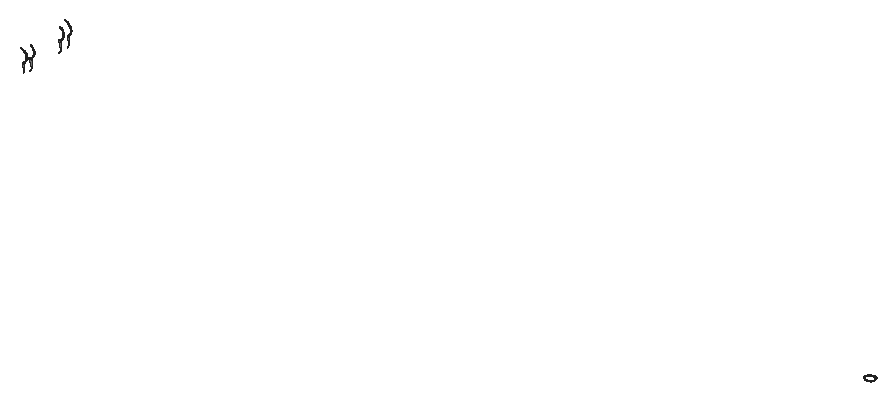
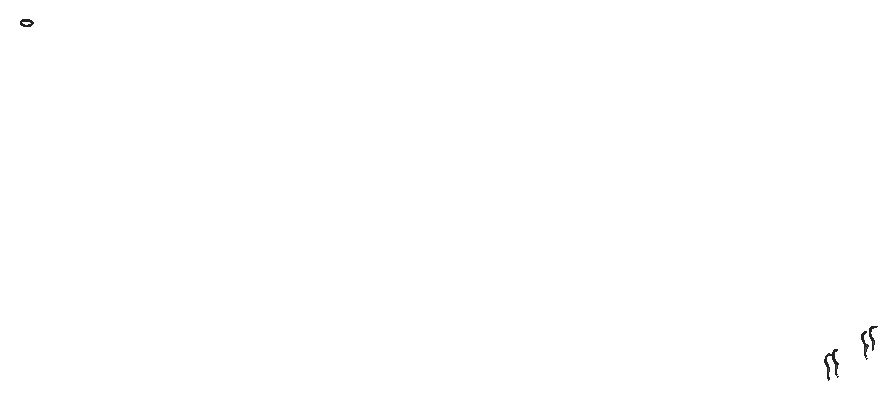
# SketchUp Ruby script. Lengths in inches.
U = 1.inch
M = Sketchup.active_model
def pt(a) = Geom::Point3d.new(a.map { |v| v * U })
def face(e, loops, mat)
  f = e.add_face(loops[0].map { |a| pt(a) })
  loops[1..].each { |l| e.add_face(l.map { |a| pt(a) }).erase! }
  f.material = f.back_material = mat if mat
  f
end
# faces: each face lists its corners as indices into pts; further lists are holes
def faces(e, pts, list, mat = nil) = list.each { |f| face(e, (f[0].is_a?(Array) ? f : [f]).map { |l| l.map { |i| pts[i] } }, mat) }
# xy, xz, yz: faces in a plane at the given z, y or x. An outline is a flat list of corners, or four numbers for a rectangle; further outlines are holes
def ring(l) = l.size == 4 ? [[l[0], l[1]], [l[2], l[1]], [l[2], l[3]], [l[0], l[3]]] : l.each_slice(2).to_a
def flat(e, list, mat, &to3) = list.each { |f| face(e, (f[0].is_a?(Array) ? f : [f]).map { |l| ring(l).map { |u, v| to3.(u, v) } }, mat) }
def xy(e, z, list, mat = nil) = flat(e, list, mat) { |x, y| [x, y, z] }
def xz(e, y, list, mat = nil) = flat(e, list, mat) { |x, z| [x, y, z] }
def yz(e, x, list, mat = nil) = flat(e, list, mat) { |y, z| [x, y, z] }
def lines(e, pts, list) = list.each { |a, b| e.add_line(pt(pts[a]), pt(pts[b])) }
# prism: a flat outline (further loops are holes) pulled along v
def prism(e, loops, v, mat = nil)
  f = face(e, loops, mat); d = Geom::Vector3d.new(v.map { |x| x * U })
  f.pushpull(f.normal.samedirection?(d) ? d.length : -d.length)
end
def box(e, o, s, mat = nil) = prism(e, [[o, [o[0] + s[0], o[1], o[2]], [o[0] + s[0], o[1] + s[1], o[2]], [o[0], o[1] + s[1], o[2]]]], [0, 0, s[2]], mat)
def at(x, y, z, deg = 0) = Geom::Transformation.translation(pt([x, y, z])) * Geom::Transformation.rotation(ORIGIN, Z_AXIS, deg.degrees)
def axes(o, x, y, z) = Geom::Transformation.new([*x, 0, *y, 0, *z, 0, *pt(o).to_a, 1])
def part(name) = M.definitions.add(name)
# library, detail: a bought-in or finely detailed component or shape, given as its bounding box
def library(name, o, s) = part(name).tap { |d| box(d.entities, o, s) }
def detail(e, o, s) = box(e.add_group.entities, o, s)
def put(e, d, t, mat = nil) = e.add_instance(d, t).tap { |i| i.material = mat if mat }
def group(e, t, mat = nil) = e.add_group.tap { |g| g.transformation = t; g.material = mat if mat }.entities
root = M.entities
M.materials.add("Material \#1").color = [140, 140, 140]
xy(root,30.4774,[[371.2232,117.1275,371.1558,117.1498,371.1662,117.166],[371.2232,117.1275,371.1662,117.166,371.2268,117.146],[371.2232,117.1275,371.2268,117.146,371.2948,117.1275],[371.2948,117.1275,371.2268,117.146,371.2912,117.146],[371.2948,117.1275,371.2912,117.146,371.3622,117.1498],
  [371.2912,117.146,371.3518,117.166,371.3622,117.1498],[371.1558,117.1498,371.101,117.1917,371.1168,117.2037],[371.1558,117.1498,371.1168,117.2037,371.1662,117.166],[371.3622,117.1498,371.3518,117.166,371.417,117.1917],[371.3518,117.166,371.4012,117.2037,371.417,117.1917],
  [371.101,117.1917,371.0651,117.2481,371.0845,117.2545],[371.101,117.1917,371.0845,117.2545,371.1168,117.2037],[371.417,117.1917,371.4012,117.2037,371.4529,117.2481],[371.4012,117.2037,371.4335,117.2545,371.4529,117.2481],[371.0651,117.2481,371.0527,117.3122,371.0733,117.3122],
  [371.0651,117.2481,371.0733,117.3122,371.0845,117.2545],[371.4529,117.2481,371.4335,117.2545,371.4653,117.3122],[371.4335,117.2545,371.4447,117.3122,371.4653,117.3122],[371.0527,117.3122,371.0651,117.3764,371.0845,117.37],[371.0527,117.3122,371.0845,117.37,371.0733,117.3122],
  [371.4447,117.3122,371.4335,117.37,371.4529,117.3764],[371.4447,117.3122,371.4529,117.3764,371.4653,117.3122],[371.0845,117.37,371.0651,117.3764,371.1168,117.4207],[371.4335,117.37,371.4012,117.4207,371.417,117.4328],[371.4335,117.37,371.417,117.4328,371.4529,117.3764],
  [371.0651,117.3764,371.101,117.4328,371.1168,117.4207],[371.1168,117.4207,371.101,117.4328,371.1662,117.4584],[371.4012,117.4207,371.3518,117.4584,371.3622,117.4746],[371.4012,117.4207,371.3622,117.4746,371.417,117.4328],[371.101,117.4328,371.1558,117.4746,371.1662,117.4584],
  [371.1662,117.4584,371.1558,117.4746,371.2268,117.4785],[371.3518,117.4584,371.2912,117.4784,371.2948,117.4969],[371.3518,117.4584,371.2948,117.4969,371.3622,117.4746],[371.1558,117.4746,371.2232,117.4969,371.2268,117.4785],[371.2912,117.4784,371.2232,117.4969,371.2948,117.4969],
  [371.2912,117.4784,371.2268,117.4785,371.2232,117.4969]],"Material \#1")
xy(root,30.4945,[[371.2232,117.1275,371.2268,117.146,371.1558,117.1498],[371.2232,117.1275,371.2912,117.146,371.2268,117.146],[371.2232,117.1275,371.2948,117.1275,371.2912,117.146],[371.2948,117.1275,371.3518,117.166,371.2912,117.146],[371.2948,117.1275,371.3622,117.1498,371.3518,117.166],
  [371.2268,117.146,371.1662,117.166,371.1558,117.1498],[371.1558,117.1498,371.1662,117.166,371.101,117.1917],[371.3622,117.1498,371.4012,117.2037,371.3518,117.166],[371.3622,117.1498,371.417,117.1917,371.4012,117.2037],[371.1662,117.166,371.1168,117.2037,371.101,117.1917],
  [371.101,117.1917,371.1168,117.2037,371.0651,117.2481],[371.417,117.1917,371.4335,117.2545,371.4012,117.2037],[371.417,117.1917,371.4529,117.2481,371.4335,117.2545],[371.1168,117.2037,371.0845,117.2545,371.0651,117.2481],[371.0651,117.2481,371.0845,117.2545,371.0527,117.3122],
  [371.4529,117.2481,371.4447,117.3122,371.4335,117.2545],[371.4529,117.2481,371.4653,117.3122,371.4447,117.3122],[371.0845,117.2545,371.0733,117.3122,371.0527,117.3122],[371.0527,117.3122,371.0733,117.3122,371.0651,117.3764],[371.0733,117.3122,371.0845,117.37,371.0651,117.3764],
  [371.4447,117.3122,371.4653,117.3122,371.4335,117.37],[371.4653,117.3122,371.4529,117.3764,371.4335,117.37],[371.0845,117.37,371.101,117.4328,371.0651,117.3764],[371.0845,117.37,371.1168,117.4207,371.101,117.4328],[371.4335,117.37,371.4529,117.3764,371.4012,117.4207],
  [371.4529,117.3764,371.417,117.4328,371.4012,117.4207],[371.1168,117.4207,371.1558,117.4746,371.101,117.4328],[371.1168,117.4207,371.1662,117.4584,371.1558,117.4746],[371.4012,117.4207,371.417,117.4328,371.3518,117.4584],[371.417,117.4328,371.3622,117.4746,371.3518,117.4584],
  [371.1662,117.4584,371.2232,117.4969,371.1558,117.4746],[371.1662,117.4584,371.2268,117.4785,371.2232,117.4969],[371.3518,117.4584,371.3622,117.4746,371.2912,117.4784],[371.3622,117.4746,371.2948,117.4969,371.2912,117.4784],[371.2912,117.4784,371.2948,117.4969,371.2268,117.4785],
  [371.2268,117.4785,371.2948,117.4969,371.2232,117.4969]],"Material \#1")
xz(root,116.5245,[[337.3754,30.1018,337.3274,30.4499,337.3734,30.4803],[337.3754,30.1018,337.3734,30.4803,337.3754,30.4138],[337.3754,30.4138,337.3734,30.4803,337.377,30.4275],[337.3754,30.4138,337.377,30.4275,337.3758,30.421],[337.377,30.4275,337.3734,30.4803,337.4118,30.5202],
  [337.377,30.4275,337.3818,30.4392,337.379,30.4336],[337.377,30.4275,337.4118,30.5202,337.3818,30.4392],[337.3818,30.4392,337.4118,30.5202,337.441,30.5681],[337.3818,30.4392,337.441,30.5681,337.4967,30.6428],[337.3818,30.4392,337.4967,30.6428,337.3853,30.4445],
  [337.3853,30.4445,337.4967,30.6428,337.3895,30.4495],[337.3895,30.4495,337.4424,30.5078,337.3945,30.4544],[337.3895,30.4495,337.4967,30.6428,337.4424,30.5078],[337.3945,30.4544,337.4424,30.5078,337.4198,30.4797],[337.4424,30.5078,337.4775,30.5711,337.4618,30.5383],
  [337.4424,30.5078,337.4967,30.6428,337.4775,30.5711],[337.441,30.5681,337.4596,30.6223,337.4967,30.6428],[337.4775,30.5711,337.4967,30.6428,337.4893,30.606],[337.4596,30.6223,337.4662,30.6813,337.4967,30.6428],[337.4967,30.6428,337.4375,30.8638,337.4918,30.7482],
  [337.4967,30.6428,337.441,30.7945,337.4375,30.8638],[337.4967,30.6428,337.4596,30.7403,337.441,30.7945],[337.4967,30.6428,337.4662,30.6813,337.4596,30.7403],[337.4967,30.6428,337.4918,30.7482,337.4992,30.6813],[337.4918,30.7482,337.4375,30.8638,337.4707,30.8096],
  [337.441,30.7945,337.4118,30.8424,337.4375,30.8638],[337.4118,30.8424,337.3734,30.8823,337.4375,30.8638],[337.4375,30.8638,337.2186,30.9732,337.3419,30.9435],[337.4375,30.8638,337.3734,30.8823,337.3274,30.9127],[337.4375,30.8638,337.3419,30.9435,337.394,30.9091]],"Material \#1")
xz(root,116.8996,[[337.2875,29.9552,337.3409,29.9997,337.3713,30.0644],[337.3409,29.9997,337.3595,30.03,337.3713,30.0644],[337.3754,30.1018,337.3754,30.4138,337.2753,30.4305],[337.3754,30.4138,337.377,30.4275,337.2753,30.4305],[337.3754,30.4138,337.3758,30.421,337.377,30.4275],
  [337.377,30.4275,337.3818,30.4392,337.2753,30.4305],[337.377,30.4275,337.379,30.4336,337.3818,30.4392],[337.3818,30.4392,337.3734,30.4803,337.3274,30.4499],[337.3818,30.4392,337.4118,30.5202,337.3734,30.4803],[337.3818,30.4392,337.3853,30.4445,337.4967,30.6428],
  [337.3818,30.4392,337.4967,30.6428,337.4118,30.5202],[337.3853,30.4445,337.3895,30.4495,337.4967,30.6428],[337.3895,30.4495,337.3945,30.4544,337.4424,30.5078],[337.3895,30.4495,337.4424,30.5078,337.4967,30.6428],[337.3945,30.4544,337.4198,30.4797,337.4424,30.5078],
  [337.4424,30.5078,337.4618,30.5383,337.4775,30.5711],[337.4424,30.5078,337.4775,30.5711,337.4967,30.6428],[337.4118,30.5202,337.4967,30.6428,337.441,30.5681],[337.441,30.5681,337.4967,30.6428,337.4596,30.6223],[337.4775,30.5711,337.4893,30.606,337.4967,30.6428],
  [337.4596,30.6223,337.4967,30.6428,337.4662,30.6813],[337.4967,30.6428,337.4375,30.8638,337.4596,30.7403],[337.4967,30.6428,337.4918,30.7482,337.4375,30.8638],[337.4967,30.6428,337.4596,30.7403,337.4662,30.6813],[337.4967,30.6428,337.4992,30.6813,337.4918,30.7482],
  [337.4596,30.7403,337.4375,30.8638,337.441,30.7945],[337.4918,30.7482,337.4707,30.8096,337.4375,30.8638],[337.441,30.7945,337.4375,30.8638,337.4118,30.8424],[337.4118,30.8424,337.4375,30.8638,337.3734,30.8823],[337.4375,30.8638,337.3274,30.9127,337.3734,30.8823],
  [337.4375,30.8638,337.394,30.9091,337.3419,30.9435]],"Material \#1")
xz(root,118.4,[[337.2875,29.9552,337.3713,30.0644,337.3409,29.9997],[337.3409,29.9997,337.3713,30.0644,337.3595,30.03],[337.3754,30.1018,337.2753,30.4305,337.3754,30.4138],[337.3754,30.4138,337.2753,30.4305,337.377,30.4275],[337.3754,30.4138,337.377,30.4275,337.3758,30.421],
  [337.377,30.4275,337.2753,30.4305,337.3818,30.4392],[337.377,30.4275,337.3818,30.4392,337.379,30.4336],[337.3818,30.4392,337.3274,30.4499,337.3734,30.4803],[337.3818,30.4392,337.3734,30.4803,337.4118,30.5202],[337.3818,30.4392,337.4118,30.5202,337.4967,30.6428],
  [337.3818,30.4392,337.4967,30.6428,337.3853,30.4445],[337.3853,30.4445,337.4967,30.6428,337.3895,30.4495],[337.3895,30.4495,337.4424,30.5078,337.3945,30.4544],[337.3895,30.4495,337.4967,30.6428,337.4424,30.5078],[337.3945,30.4544,337.4424,30.5078,337.4198,30.4797],
  [337.4424,30.5078,337.4775,30.5711,337.4618,30.5383],[337.4424,30.5078,337.4967,30.6428,337.4775,30.5711],[337.4118,30.5202,337.441,30.5681,337.4967,30.6428],[337.441,30.5681,337.4596,30.6223,337.4967,30.6428],[337.4775,30.5711,337.4967,30.6428,337.4893,30.606],
  [337.4596,30.6223,337.4662,30.6813,337.4967,30.6428],[337.4967,30.6428,337.4375,30.8638,337.4918,30.7482],[337.4967,30.6428,337.4596,30.7403,337.4375,30.8638],[337.4967,30.6428,337.4662,30.6813,337.4596,30.7403],[337.4967,30.6428,337.4918,30.7482,337.4992,30.6813],
  [337.4596,30.7403,337.441,30.7945,337.4375,30.8638],[337.4918,30.7482,337.4375,30.8638,337.4707,30.8096],[337.441,30.7945,337.4118,30.8424,337.4375,30.8638],[337.4118,30.8424,337.3734,30.8823,337.4375,30.8638],[337.4375,30.8638,337.3734,30.8823,337.3274,30.9127],
  [337.4375,30.8638,337.3419,30.9435,337.394,30.9091]],"Material \#1")
xz(root,118.7751,[[337.3409,29.9997,337.3595,30.03,337.3713,30.0644],[337.3409,29.9997,337.3713,30.0644,337.3754,30.1018],[337.3754,30.1018,337.3734,30.4803,337.3274,30.4499],[337.3754,30.1018,337.3754,30.4138,337.3734,30.4803],[337.3754,30.4138,337.377,30.4275,337.3734,30.4803],
  [337.3754,30.4138,337.3758,30.421,337.377,30.4275],[337.377,30.4275,337.4118,30.5202,337.3734,30.4803],[337.377,30.4275,337.379,30.4336,337.3818,30.4392],[337.377,30.4275,337.3818,30.4392,337.4118,30.5202],[337.3818,30.4392,337.3853,30.4445,337.4967,30.6428],
  [337.3818,30.4392,337.441,30.5681,337.4118,30.5202],[337.3818,30.4392,337.4967,30.6428,337.441,30.5681],[337.3853,30.4445,337.3895,30.4495,337.4967,30.6428],[337.3895,30.4495,337.3945,30.4544,337.4424,30.5078],[337.3895,30.4495,337.4424,30.5078,337.4967,30.6428],
  [337.3945,30.4544,337.4198,30.4797,337.4424,30.5078],[337.4424,30.5078,337.4618,30.5383,337.4775,30.5711],[337.4424,30.5078,337.4775,30.5711,337.4967,30.6428],[337.441,30.5681,337.4967,30.6428,337.4596,30.6223],[337.4775,30.5711,337.4893,30.606,337.4967,30.6428],
  [337.4596,30.6223,337.4967,30.6428,337.4662,30.6813],[337.4967,30.6428,337.4375,30.8638,337.441,30.7945],[337.4967,30.6428,337.4918,30.7482,337.4375,30.8638],[337.4967,30.6428,337.441,30.7945,337.4596,30.7403],[337.4967,30.6428,337.4596,30.7403,337.4662,30.6813],
  [337.4967,30.6428,337.4992,30.6813,337.4918,30.7482],[337.4918,30.7482,337.4707,30.8096,337.4375,30.8638],[337.441,30.7945,337.4375,30.8638,337.4118,30.8424],[337.4118,30.8424,337.4375,30.8638,337.3734,30.8823],[337.4375,30.8638,337.3419,30.9435,337.2186,30.9732],
  [337.4375,30.8638,337.3274,30.9127,337.3734,30.8823],[337.4375,30.8638,337.394,30.9091,337.3419,30.9435]],"Material \#1")
